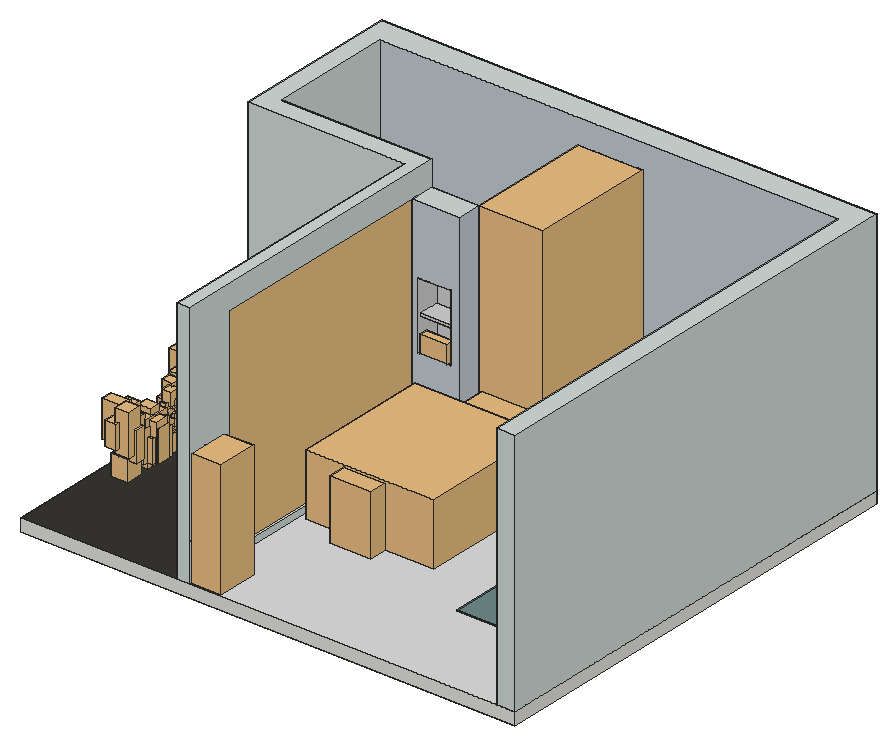
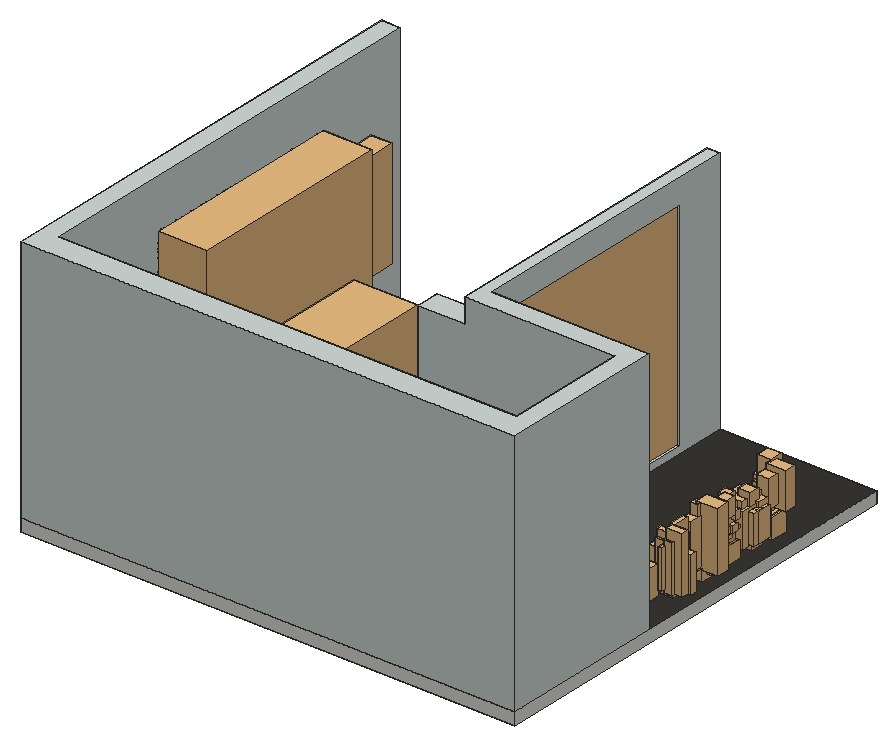
# SketchUp Ruby script. Lengths in inches.
U = 1.inch
M = Sketchup.active_model
def pt(a) = Geom::Point3d.new(a.map { |v| v * U })
def face(e, loops, mat)
  f = e.add_face(loops[0].map { |a| pt(a) })
  loops[1..].each { |l| e.add_face(l.map { |a| pt(a) }).erase! }
  f.material = f.back_material = mat if mat
  f
end
# faces: each face lists its corners as indices into pts; further lists are holes
def faces(e, pts, list, mat = nil) = list.each { |f| face(e, (f[0].is_a?(Array) ? f : [f]).map { |l| l.map { |i| pts[i] } }, mat) }
# xy, xz, yz: faces in a plane at the given z, y or x. An outline is a flat list of corners, or four numbers for a rectangle; further outlines are holes
def ring(l) = l.size == 4 ? [[l[0], l[1]], [l[2], l[1]], [l[2], l[3]], [l[0], l[3]]] : l.each_slice(2).to_a
def flat(e, list, mat, &to3) = list.each { |f| face(e, (f[0].is_a?(Array) ? f : [f]).map { |l| ring(l).map { |u, v| to3.(u, v) } }, mat) }
def xy(e, z, list, mat = nil) = flat(e, list, mat) { |x, y| [x, y, z] }
def xz(e, y, list, mat = nil) = flat(e, list, mat) { |x, z| [x, y, z] }
def yz(e, x, list, mat = nil) = flat(e, list, mat) { |y, z| [x, y, z] }
def lines(e, pts, list) = list.each { |a, b| e.add_line(pt(pts[a]), pt(pts[b])) }
# prism: a flat outline (further loops are holes) pulled along v
def prism(e, loops, v, mat = nil)
  f = face(e, loops, mat); d = Geom::Vector3d.new(v.map { |x| x * U })
  f.pushpull(f.normal.samedirection?(d) ? d.length : -d.length)
end
def box(e, o, s, mat = nil) = prism(e, [[o, [o[0] + s[0], o[1], o[2]], [o[0] + s[0], o[1] + s[1], o[2]], [o[0], o[1] + s[1], o[2]]]], [0, 0, s[2]], mat)
def at(x, y, z, deg = 0) = Geom::Transformation.translation(pt([x, y, z])) * Geom::Transformation.rotation(ORIGIN, Z_AXIS, deg.degrees)
def axes(o, x, y, z) = Geom::Transformation.new([*x, 0, *y, 0, *z, 0, *pt(o).to_a, 1])
def part(name) = M.definitions.add(name)
# library, detail: a bought-in or finely detailed component or shape, given as its bounding box
def library(name, o, s) = part(name).tap { |d| box(d.entities, o, s) }
def detail(e, o, s) = box(e.add_group.entities, o, s)
def put(e, d, t, mat = nil) = e.add_instance(d, t).tap { |i| i.material = mat if mat }
def group(e, t, mat = nil) = e.add_group.tap { |g| g.transformation = t; g.material = mat if mat }.entities
root = M.entities
M.materials.add("1467 AP 9475 Shining Blue").color = [208, 218, 214]
M.materials.add("BANANA_BIG_STVOL_1").color = [93, 83, 53]
M.materials.add("Goldfish-custom-shape__54193.1487305638").color = [111, 138, 137]
M.materials.add("POT_TEXTURE_1").color = [172, 172, 172]
M.materials.add("POT_TEXTURE_2").color = [160, 154, 144]
M.materials.add("[Carrera Marble]").color = [207, 207, 207]
M.materials.add("[Marble Carrara Gold Floor Tile]").color = [221, 221, 221]
M.materials.add("[Metal Seamed]").color = [67, 65, 65]
M.materials.add("[Stone Brushed Khaki]").color = [196, 204, 211]
M.materials.add("[Tile Travertine 2 inch]").color = [56, 54, 50]
M.materials.add("[Translucent Glass Blue]").color = [192, 204, 226]
M.materials["[Translucent Glass Blue]"].alpha = 0.5
M.materials.add("[Wood Floor]").color = [107, 58, 35]
M.materials.add("soil1").color = [68, 55, 47]
M.materials.add("white_concrete_pot1").color = [212, 211, 204]
M.materials.add("wood_1").color = [140, 119, 94]
c1 = library("Сауна. Дренаж",[0,0,0],[36,3.67,1.375])
c2 = library("plant\#1",[-21.34,-27.21,-0.38],[41.91,41.15,38.97])
c3 = library("Untitled",[118.83,25.61,-0.38],[19.68,14.54,56.29])
c4 = library("Group\#283",[-640.625,-1318.37,287.11],[396.64,314.81,689.96])
c5 = library("Group\#277",[-513.94,-1201.2,195.17],[480.66,557.42,1160.08])
c6 = library("Group\#279",[-208.03,-1336.63,286.21],[381.72,484.79,1145.39])
c7 = library("Group\#286",[-619.83,-1636.3,288.9],[316.15,456.61,1171.28])
c8 = library("Group\#287",[-738.91,-1210.08,301],[426.4,388.88,1000.79])
c9 = library("Group\#289",[-208.33,-1511.76,297.04],[508.2,421.96,1258.76])
c10 = library("Group\#278",[-545.36,-1775.03,287.125],[412.21,432,920.68])
c11 = library("Group\#284",[-750.24,-1478.51,301.56],[423.84,451.05,998.69])
c12 = library("Group\#282",[-245.33,-1174.2,301.22],[356.02,306.31,608.34])
c13 = library("Group\#276",[-487.23,-1483.58,-4.71],[450.86,446.99,418.38])
c14 = library("Group\#291",[-445.7,-1606.55,154.18],[255.44,283.57,849.28])
c15 = library("Group\#292",[-390.1,-1177.12,195.59],[220.93,265.44,790.12])
c16 = library("Group\#294",[-480.32,-1333.42,295.8],[424.49,356.06,1482.77])
c17 = library("Group\#295",[-378.01,-1245.98,305.66],[422.15,474.55,1267.42])
c18 = library("Group\#281",[-163.65,-1622.09,292.29],[406.18,374.8,780.12])
c19 = library("Group\#290",[-384.8,-1640.99,300.61],[422.68,348.03,1297.96])
c20 = library("Group\#275",[-429.18,-1441.17,362.05],[345.84,348.28,45.35])
c21 = library("Group\#293",[-208.0625,-1498.77,286.27],[547.26,435.76,1075.6])
c22 = library("Group\#288",[-172.82,-1329.68,294.68],[502.85,397.72,955.79])
c23 = library("Group\#285",[-426.76,-1753.59,287.48],[479.67,412.35,1049.19])
c24 = part("Potted palm")
put(c24.entities,c4,at(750.24,1775.03,4.71))
put(c24.entities,c5,at(750.24,1775.03,4.71))
put(c24.entities,c6,at(750.24,1775.03,4.71))
put(c24.entities,c7,at(750.24,1775.03,4.71))
put(c24.entities,c8,at(750.24,1775.03,4.71))
put(c24.entities,c9,at(750.24,1775.03,4.71))
put(c24.entities,c10,at(750.24,1775.03,4.71))
put(c24.entities,c11,at(750.24,1775.03,4.71))
put(c24.entities,c12,at(750.24,1775.03,4.71))
put(c24.entities,c13,at(750.24,1775.03,4.71),"POT_TEXTURE_1")
put(c24.entities,c14,at(750.24,1775.03,4.71))
put(c24.entities,c15,at(750.24,1775.03,4.71))
put(c24.entities,c16,at(750.24,1775.03,4.71))
put(c24.entities,c17,at(750.24,1775.03,4.71))
put(c24.entities,c18,at(750.24,1775.03,4.71))
put(c24.entities,c19,at(750.24,1775.03,4.71))
put(c24.entities,c20,at(750.24,1775.03,4.71),"soil1")
put(c24.entities,c21,at(750.24,1775.03,4.71))
put(c24.entities,c22,at(750.24,1775.03,4.71))
put(c24.entities,c23,at(750.24,1775.03,4.71))
c25 = library("Scara cu plante",[-7.66,-9.41,-0.15],[30.59,22.83,66.38])
c26 = library("bain4",[0,0,0],[65.98,62.12,30.23])
c27 = library("Group\#14",[0,0,0],[31.13,60.5,108])
c28 = library("Wall hung toilet",[0.42,0,0],[26.94,19.69,42.125])
c29 = part("Goldfish Aqua Runner")
box(c29.entities,[0,0,0],[43.79,100,0.375],"Goldfish-custom-shape__54193.1487305638")
c30 = library("Bathroom Stool and Styling",[15.82,12.47,0],[25.92,25.93,28.18])
c31 = part("Group228\#1")
box(c31.entities,[-18,-24,0],[36,5,0.25])
c32 = part("Group229\#1")
box(c32.entities,[-18,-18.5,0],[36,5,0.25])
c33 = part("Group230\#1")
box(c33.entities,[-18,-13,0],[36,5,0.25])
c34 = part("Group231\#1")
box(c34.entities,[-18,-7.5,0],[36,5,0.25])
c35 = part("Group232\#1")
box(c35.entities,[-18,-2,0],[36,5,0.25])
c36 = part("Group233\#1")
box(c36.entities,[-18,3.5,0],[36,5,0.25])
c37 = part("Group234\#1")
box(c37.entities,[-18,9,0],[36,5,0.25])
c38 = part("Group235\#1")
box(c38.entities,[-18,14.5,0],[36,5,0.25])
c39 = part("Group236\#1")
box(c39.entities,[-18,20,0],[36,4,0.25])
c40 = part("Group226\#1")
put(c40.entities,c31,at(0,0,0))
put(c40.entities,c32,at(0,0,0))
put(c40.entities,c33,at(0,0,0))
put(c40.entities,c34,at(0,0,0))
put(c40.entities,c35,at(0,0,0))
put(c40.entities,c36,at(0,0,0))
put(c40.entities,c37,at(0,0,0))
put(c40.entities,c38,at(0,0,0))
put(c40.entities,c39,at(0,0,0))
c41 = library("Bathroom stool",[0,0,0],[19.9375,11.76,29.04])
c42 = library("Plant\#2",[0,0,0],[12.59,12.59,14.16])
c43 = library("Group\#242",[-662.41,217.3,320.04],[397.32,658.3,1732.06])
c44 = library("Group\#244",[-299.2,181.55,262.58],[360.65,735.71,1258.34])
c45 = library("Group\#239",[-1038.76,656.55,345.34],[733.18,460.51,2065.7])
c46 = library("Group\#237",[-445.29,890.31,329.28],[284.3,304.08,2023.29])
c47 = library("Group\#240",[-733.48,439.625,202.64],[456.28,533.12,1536.78])
c48 = library("Group\#243",[-455.56,899.32,410.78],[341.21,610.33,1581.5])
c49 = library("Group\#236",[-516.34,626.77,-4.5625],[517.73,515.95,418.98])
c50 = library("Group\#241",[-249.24,914.85,310.18],[345.55,647.95,1307.93])
c51 = library("Group\#238",[-277.97,488.68,287.26],[362.84,405.94,1768.54])
c52 = library("Group\#235",[-468.76,669.89,380.1875],[424.36,427.47,41.99])
c53 = part("Potted tropical plant")
put(c53.entities,c43,at(1038.76,-181.55,4.5625))
put(c53.entities,c44,at(1038.76,-181.55,4.5625))
put(c53.entities,c45,at(1038.76,-181.55,4.5625))
put(c53.entities,c46,at(1038.76,-181.55,4.5625))
put(c53.entities,c47,at(1038.76,-181.55,4.5625))
put(c53.entities,c48,at(1038.76,-181.55,4.5625))
put(c53.entities,c49,at(1038.76,-181.55,4.5625),"POT_TEXTURE_1")
put(c53.entities,c50,at(1038.76,-181.55,4.5625))
put(c53.entities,c51,at(1038.76,-181.55,4.5625))
put(c53.entities,c52,at(1038.76,-181.55,4.5625),"soil1")
c54 = library("Group\#248",[-246.45,-349.05,558.47],[136.91,100.49,66.1])
c55 = library("Group\#251",[-264.68,-415.73,1484.11],[304.64,209.69,227.41])
c56 = library("Group\#259",[-357.04,-394.18,1447.05],[213.62,306.36,356.95])
c57 = library("Group\#246",[-447.02,-464.95,536.35],[343.73,346.24,39.39])
c58 = library("Group\#247",[-394.9,-448.99,911.74],[90.19,96.88,85.93])
c59 = library("Group\#258",[-424,-312.27,817.53],[158.81,108.06,136.45])
c60 = library("Group\#262",[-409.02,-515.05,915.53],[69.62,77.27,65.47])
c61 = library("Group\#266",[-548.25,-262.82,1459.54],[373.26,352.35,568])
c62 = library("Group\#274",[-492.14,-508.4,-4.15],[433.72,431.71,567.03])
c63 = library("Group\#269",[-293.78,-482.77,597.9],[158.75,112.78,159.87])
c64 = library("Group\#252",[-545.09,-386.51,922.3125],[300.25,219.65,227.33])
c65 = library("Group\#271",[-292.81,-667.38,1418.14],[215.17,356.07,188.87])
c66 = library("Group\#254",[-292.14,-288.9,1281.79],[169.55,204.34,203.36])
c67 = library("Group\#260",[-568.91,-444.37,1285.4],[307.6,179.39,277.93])
c68 = library("Group\#257",[-341.93,-403.49,744.8125],[64.83,96.32,132.15])
c69 = library("Group\#245",[-258.04,-282.68,604.05],[115.53,137.01,52.63])
c70 = library("Group\#253",[-304.79,-269.16,622.65],[82.06,111.89,102.57])
c71 = library("Group\#261",[-388.93,-514.39,838.93],[89.79,77.73,82.08])
c72 = library("Group\#263",[-295.03,-516.52,742.34],[68.71,141.75,78.67])
c73 = library("Group\#270",[-422.77,-235.4,843.61],[178.54,197.77,233.54])
c74 = library("Group\#264",[-498.98,-524.4,908.45],[120.83,107.95,112.98])
c75 = library("Group\#267",[-321.08,-139.66,1308.49],[285.55,393.29,221.53])
c76 = library("Group\#265",[-278.4,-571.99,1530.91],[311.57,345.77,423.62])
c77 = library("Group\#268",[-387.74,-136.11,1470.07],[230,321.58,230.27])
c78 = library("Group\#256",[-244.55,-305.59,1009.46],[103.13,76.81,77.34])
c79 = library("Group\#273",[-385.21,-446.52,494.02],[160.93,321.12,1142.36])
c80 = library("Group\#249",[-249.18,-250.59,980.93],[152.21,116.16,134.05])
c81 = library("Group\#250",[-438.92,-265.61,702.3],[171.52,146.16,133.5])
c82 = part("Potted houseplant")
p = [[568.91,667.38,4.15],[569.91,667.38,4.15],[569.91,668.38,4.15]]
lines(c82.entities,p,[[0,1],[1,2],[2,0]])
put(c82.entities,c54,at(568.91,667.38,4.15))
put(c82.entities,c55,at(568.91,667.38,4.15))
put(c82.entities,c56,at(568.91,667.38,4.15))
put(c82.entities,c57,at(568.91,667.38,4.15),"soil1")
put(c82.entities,c58,at(568.91,667.38,4.15))
put(c82.entities,c59,at(568.91,667.38,4.15))
put(c82.entities,c60,at(568.91,667.38,4.15))
put(c82.entities,c61,at(568.91,667.38,4.15))
put(c82.entities,c62,at(568.91,667.38,4.15),"POT_TEXTURE_2")
put(c82.entities,c63,at(568.91,667.38,4.15))
put(c82.entities,c64,at(568.91,667.38,4.15))
put(c82.entities,c65,at(568.91,667.38,4.15))
put(c82.entities,c66,at(568.91,667.38,4.15))
put(c82.entities,c67,at(568.91,667.38,4.15))
put(c82.entities,c68,at(568.91,667.38,4.15))
put(c82.entities,c69,at(568.91,667.38,4.15))
put(c82.entities,c70,at(568.91,667.38,4.15))
put(c82.entities,c71,at(568.91,667.38,4.15))
put(c82.entities,c72,at(568.91,667.38,4.15))
put(c82.entities,c73,at(568.91,667.38,4.15))
put(c82.entities,c74,at(568.91,667.38,4.15))
put(c82.entities,c75,at(568.91,667.38,4.15))
put(c82.entities,c76,at(568.91,667.38,4.15))
put(c82.entities,c77,at(568.91,667.38,4.15))
put(c82.entities,c78,at(568.91,667.38,4.15))
put(c82.entities,c79,at(568.91,667.38,4.15),"wood_1")
put(c82.entities,c80,at(568.91,667.38,4.15))
put(c82.entities,c81,at(568.91,667.38,4.15))
c83 = library("Group\#296",[-480.3,-2300.47,677.45],[398.14,398.43,28.25])
c84 = library("Group\#297",[-336.38,-2175.79,614.41],[133.99,147.1,560.64])
c85 = library("Group\#298",[-311.45,-2362.85,663.67],[597.01,322.07,1007.38])
c86 = library("Group\#299",[-330.26,-2159.14,612.04],[116.66,119.22,673.97])
c87 = library("Group\#302",[-667.53,-2111.4375,1071.74],[420.02,555.28,968.03])
c88 = library("Group\#303",[-328.97,-2115.58,1156.29],[117.86,119.42,695.38])
c89 = library("Group\#305",[-943.22,-2312.1875,967.59],[670.63,402.45,1245.73])
c90 = library("Group\#308",[-343.93,-2076.42,1024.91],[285.05,475.82,708.21])
c91 = library("Group\#306",[-568.09,-2386.9,-3.76],[573.62,569.18,700.28])
c92 = library("Group\#309",[-550.09,-2664.39,1031.96],[371.42,533.86,798])
c93 = library("Group\#310",[-308.37,-2556.11,869.35],[483.58,483.6,1385.8])
c94 = part("Potted tropical plant \#1")
put(c94.entities,c83,at(943.22,2664.39,3.76),"soil1")
put(c94.entities,c84,at(943.22,2664.39,3.76),"BANANA_BIG_STVOL_1")
put(c94.entities,c85,at(943.22,2664.39,3.76))
put(c94.entities,c86,at(943.22,2664.39,3.76),"BANANA_BIG_STVOL_1")
put(c94.entities,c87,at(943.22,2664.39,3.76))
put(c94.entities,c88,at(943.22,2664.39,3.76))
put(c94.entities,c89,at(943.22,2664.39,3.76))
put(c94.entities,c90,at(943.22,2664.39,3.76))
put(c94.entities,c91,at(943.22,2664.39,3.76),"POT_TEXTURE_2")
put(c94.entities,c92,at(943.22,2664.39,3.76))
put(c94.entities,c93,at(943.22,2664.39,3.76))
c95 = library("Group\#119",[-312.76,2118.02,370.79],[80.37,61.43,57.53])
c96 = library("Group\#164",[-146.29,2044.53,349.125],[81,53.32,37.9])
c97 = library("Group\#231",[-236.03,2064.57,238.29],[378.97,266.89,1422.96])
c98 = library("Group\#132",[-392.38,2142.99,345.23],[79.77,60.6,39.05])
c99 = library("Group\#193",[-390.04,2074.71,363.78],[77.3,84.83,61.55])
c100 = library("Group\#142",[-389.63,2051.04,359.41],[56.81,81.38,37.86])
c101 = library("Group\#146",[-362.86,1963.26,351.01],[55.56,80.44,37.9])
c102 = library("Group\#163",[-200.52,1998.86,370.22],[77.15,68.38,35.39])
c103 = library("Group\#184",[-480.58,1843.32,11.96],[467.85,466.24,378.92])
c104 = library("Group\#133",[-433.57,2042.61,369.7],[71.79,72.8,37.85])
c105 = library("Group\#130",[-148.5,2084.1,354.63],[73.89,71.73,39.48])
c106 = library("Group\#205",[-372.4375,2154.5,374],[76.125,67.08,39.0625])
c107 = library("Group\#206",[-275.5,2156.34,352.11],[71.39,73.27,44.69])
c108 = library("Group\#174",[-143.56,2061.14,371.42],[79.79,63.19,51.3])
c109 = library("Group\#192",[-363.89,1895.22,354.63],[76.92,66.54,39.48])
c110 = library("Group\#176",[-145.08,2015.32,369.99],[82.29,54.05,37.9])
c111 = library("Group\#203",[-315.77,2202.04,371],[80.74,54.44,37.85])
c112 = library("Group\#194",[-419.21,1941.11,355.02],[73.1,71.21,39.06])
c113 = library("Group\#199",[-229.79,1894.04,351.01],[79.82,63.55,37.9])
c114 = library("Group\#210",[-234.26,2180.97,367.05],[50.63,74.65,43.95])
c115 = library("Group\#213",[-904.81,1865.01,156.3],[624.43,217.34,1227.7])
c116 = library("Group\#214",[-312.51,1611.52,263.78],[120.52,408.52,1275.1])
c117 = library("Group\#217",[-571.16,1736.08,232.33],[294.08,306.57,1438.75])
c118 = library("Group\#222",[-273.21,1593.22,47.51],[374.54,419.07,1416.6])
c119 = library("Group\#123",[-202.35,1900.5,372.29],[58.53,80.11,50.06])
c120 = library("Group\#135",[-432.01,1984.38,372.6875],[64.1,75.95,39.0625])
c121 = library("Group\#168",[-310.7,1952.62,354.63],[79.53,58.52,39.48])
c122 = library("Group\#134",[-374.28,1979.7,369.99],[51.81,82.66,37.9])
c123 = library("Group\#201",[-397.18,1916.74,372.44],[70.02,74.57,49.25])
c124 = library("Group\#208",[-236.3,2186.8,344.47],[79.26,62.91,39.06])
c125 = library("Group\#122",[-161.07,2117.49,373.61],[81.25,53.73,39.48])
c126 = library("Group\#212",[-431.9,1883.46,368.72],[373.65,376.39,18.61])
c127 = library("Group\#167",[-340.96,1970.4,361.28],[81.22,51.59,61.62])
c128 = library("Group\#179",[-272.7,1884.51,369.99],[80.39,55.87,37.9])
c129 = library("Group\#153",[-330.83,2117.69,370.2],[61.83,80.2,35.55])
c130 = library("Group\#209",[-366.3125,2177.8,359.41],[79.9,61.23,37.86])
c131 = library("Group\#145",[-435.875,2067.96,347.82],[58.32,80.53,38.29])
c132 = library("Group\#207",[-183.79,2161.45,371.25],[72.43,70.21,54.35])
c133 = library("Group\#221",[-208.23,2037.18,75.37],[621.09,225.61,1251.82])
c134 = library("Group\#225",[-675.58,1862.05,152.55],[378.81,196.01,1743.84])
c135 = library("Group\#226",[-257.06,2048.08,160.05],[394.6,177.93,1743.83])
c136 = library("Group\#228",[-344.84,1500.61,160.55],[176.35,551.19,1921.45])
c137 = library("Group\#229",[-231.77,1913.24,119.96],[448.93,143.84,1582.05])
c138 = library("Group\#230",[-616.67,2098.6,178.29],[331.19,111.16,1177.92])
c139 = library("Group\#223",[-527.15,2088.47,150.96],[267.01,328.12,1599.25])
c140 = library("Group\#232",[-792.12,2067.32,152.13],[549.56,259.52,1931.8])
c141 = library("Group\#234",[-281.17,2118.67,243.77],[133.23,408.71,1313.3])
c142 = part("Potted houseplant \#1")
g1 = group(c142.entities,at(904.81,-1500.61,-11.96),"white_concrete_pot1")
detail(g1,[-222.14,2117.95,372.07],[61.87,75.41,50.35])
put(c142.entities,c95,at(904.81,-1500.61,-11.96),"white_concrete_pot1")
g2 = group(c142.entities,at(904.81,-1500.61,-11.96),"white_concrete_pot1")
detail(g2,[-313.93,1881.02,351.21],[70.15,73.18,37.2])
g3 = group(c142.entities,at(904.81,-1500.61,-11.96),"white_concrete_pot1")
detail(g3,[-209.1,1970.26,378.89],[50.57,81.04,37.2])
put(c142.entities,c96,at(904.81,-1500.61,-11.96),"white_concrete_pot1")
put(c142.entities,c97,at(904.81,-1500.61,-11.96))
put(c142.entities,c98,at(904.81,-1500.61,-11.96),"white_concrete_pot1")
put(c142.entities,c99,at(904.81,-1500.61,-11.96),"white_concrete_pot1")
put(c142.entities,c100,at(904.81,-1500.61,-11.96),"white_concrete_pot1")
put(c142.entities,c101,at(904.81,-1500.61,-11.96),"white_concrete_pot1")
g4 = group(c142.entities,at(904.81,-1500.61,-11.96),"white_concrete_pot1")
detail(g4,[-129.49,1972.75,359.91],[55.59,80.76,37.2])
put(c142.entities,c102,at(904.81,-1500.61,-11.96),"white_concrete_pot1")
g5 = group(c142.entities,at(904.81,-1500.61,-11.96),"white_concrete_pot1")
detail(g5,[-333.13,1892.25,370.19],[61.39,79.4,37.2])
put(c142.entities,c103,at(904.81,-1500.61,-11.96),"POT_TEXTURE_1")
put(c142.entities,c104,at(904.81,-1500.61,-11.96),"white_concrete_pot1")
put(c142.entities,c105,at(904.81,-1500.61,-11.96),"white_concrete_pot1")
g6 = group(c142.entities,at(904.81,-1500.61,-11.96),"white_concrete_pot1")
detail(g6,[-270.91,2176.57,345.18],[52.11,82.01,38.29])
g7 = group(c142.entities,at(904.81,-1500.61,-11.96),"white_concrete_pot1")
detail(g7,[-195.71,2019.1875,371.11],[58.98,81.18,37.2])
g8 = group(c142.entities,at(904.81,-1500.61,-11.96),"white_concrete_pot1")
detail(g8,[-319.36,2078.81,339.18],[76.07,69.08,39.48])
put(c142.entities,c106,at(904.81,-1500.61,-11.96),"white_concrete_pot1")
put(c142.entities,c107,at(904.81,-1500.61,-11.96),"white_concrete_pot1")
g9 = group(c142.entities,at(904.81,-1500.61,-11.96),"white_concrete_pot1")
detail(g9,[-417.64,2112.53,369.82],[65.44,79.59,38.29])
put(c142.entities,c108,at(904.81,-1500.61,-11.96),"white_concrete_pot1")
put(c142.entities,c109,at(904.81,-1500.61,-11.96),"white_concrete_pot1")
put(c142.entities,c110,at(904.81,-1500.61,-11.96),"white_concrete_pot1")
g10 = group(c142.entities,at(904.81,-1500.61,-11.96),"white_concrete_pot1")
detail(g10,[-240.6,2054.85,378.89],[71.5,72.03,37.2])
put(c142.entities,c111,at(904.81,-1500.61,-11.96),"white_concrete_pot1")
put(c142.entities,c112,at(904.81,-1500.61,-11.96),"white_concrete_pot1")
put(c142.entities,c113,at(904.81,-1500.61,-11.96),"white_concrete_pot1")
g11 = group(c142.entities,at(904.81,-1500.61,-11.96),"white_concrete_pot1")
detail(g11,[-249.82,2117.53,359.91],[58.07,81.25,37.2])
put(c142.entities,c114,at(904.81,-1500.61,-11.96),"white_concrete_pot1")
put(c142.entities,c115,at(904.81,-1500.61,-11.96))
put(c142.entities,c116,at(904.81,-1500.61,-11.96))
put(c142.entities,c117,at(904.81,-1500.61,-11.96))
put(c142.entities,c118,at(904.81,-1500.61,-11.96))
g12 = group(c142.entities,at(904.81,-1500.61,-11.96),"white_concrete_pot1")
detail(g12,[-435.4375,2027.54,350.71],[78.74,62.6,37.86])
put(c142.entities,c119,at(904.81,-1500.61,-11.96),"white_concrete_pot1")
g13 = group(c142.entities,at(904.81,-1500.61,-11.96),"white_concrete_pot1")
detail(g13,[-173.8,2126.25,354.63],[80.17,60.53,39.48])
g14 = group(c142.entities,at(904.81,-1500.61,-11.96),"white_concrete_pot1")
detail(g14,[-222.96,2066.75,359.91],[63.77,78.21,37.2])
put(c142.entities,c120,at(904.81,-1500.61,-11.96),"white_concrete_pot1")
g15 = group(c142.entities,at(904.81,-1500.61,-11.96),"white_concrete_pot1")
detail(g15,[-183.125,1913.38,330.04],[66.78,77.69,39.48])
put(c142.entities,c121,at(904.81,-1500.61,-11.96),"white_concrete_pot1")
g16 = group(c142.entities,at(904.81,-1500.61,-11.96),"white_concrete_pot1")
detail(g16,[-152,1936.85,378.89],[64.46,79.76,37.2])
g17 = group(c142.entities,at(904.81,-1500.61,-11.96),"white_concrete_pot1")
detail(g17,[-284.65,1933.22,373.64],[80.83,55.23,37.2])
put(c142.entities,c122,at(904.81,-1500.61,-11.96),"white_concrete_pot1")
g18 = group(c142.entities,at(904.81,-1500.61,-11.96),"white_concrete_pot1")
detail(g18,[-263.49,1923.54,359.91],[75.98,66.75,37.2])
put(c142.entities,c123,at(904.81,-1500.61,-11.96),"white_concrete_pot1")
g19 = group(c142.entities,at(904.81,-1500.61,-11.96),"white_concrete_pot1")
detail(g19,[-167.97,1940.97,354.63],[66.78,77.7,39.48])
put(c142.entities,c124,at(904.81,-1500.61,-11.96),"white_concrete_pot1")
g20 = group(c142.entities,at(904.81,-1500.61,-11.96),"white_concrete_pot1")
detail(g20,[-214.75,1956.59,330.04],[66.78,77.69,39.48])
put(c142.entities,c125,at(904.81,-1500.61,-11.96),"white_concrete_pot1")
put(c142.entities,c126,at(904.81,-1500.61,-11.96),"white_concrete_pot1")
put(c142.entities,c127,at(904.81,-1500.61,-11.96),"white_concrete_pot1")
g21 = group(c142.entities,at(904.81,-1500.61,-11.96),"white_concrete_pot1")
detail(g21,[-282.5625,1934.21,389.56],[81.1,59.19,35.03])
put(c142.entities,c128,at(904.81,-1500.61,-11.96),"white_concrete_pot1")
g22 = group(c142.entities,at(904.81,-1500.61,-11.96),"white_concrete_pot1")
detail(g22,[-394.5,2036.48,359.91],[79.58,64.84,37.2])
put(c142.entities,c129,at(904.81,-1500.61,-11.96),"white_concrete_pot1")
put(c142.entities,c130,at(904.81,-1500.61,-11.96),"white_concrete_pot1")
put(c142.entities,c131,at(904.81,-1500.61,-11.96),"white_concrete_pot1")
put(c142.entities,c132,at(904.81,-1500.61,-11.96),"white_concrete_pot1")
put(c142.entities,c133,at(904.81,-1500.61,-11.96))
put(c142.entities,c134,at(904.81,-1500.61,-11.96))
put(c142.entities,c135,at(904.81,-1500.61,-11.96))
put(c142.entities,c136,at(904.81,-1500.61,-11.96))
put(c142.entities,c137,at(904.81,-1500.61,-11.96))
put(c142.entities,c138,at(904.81,-1500.61,-11.96))
put(c142.entities,c139,at(904.81,-1500.61,-11.96))
put(c142.entities,c140,at(904.81,-1500.61,-11.96))
put(c142.entities,c141,at(904.81,-1500.61,-11.96))
c143 = library("Group\#16",[-0.5,0,0],[3,114,105])
c144 = part("Group\#18")
box(c144.entities,[-0.47,0,0],[0.47,56,101])
c145 = library("Group\#5",[-20.5,-2,0],[20.5,100,87])
c146 = library("Wall Tap 1",[0,0,0],[12.6,7.22,3.6875])
c147 = library("JEE-O slimline shower set bronze\#1",[0.04,-0.03,-18.98],[11.61,24.11,65.69])
c148 = library("Bathrobe with hooks",[0,0,-0.08],[18.125,10.02,52.34])
c149 = library("Group\#52",[0,-0.31,0],[12.93,3.92,8.58])
xy(root,0,[[76,0,76,138,0,138,0,219,240,219,240,0,231,0,231,147,195,147,195,153,231,153,231,207,9,207,9,147,105,147,105,135,82,135,82,0]],"1467 AP 9475 Shining Blue")
xy(root,3,[[76,24,82,138]],"1467 AP 9475 Shining Blue")
xy(root,42,[[85,135,101,146]],"[Carrera Marble]")
xy(root,48,[[195,147,231,153]],"1467 AP 9475 Shining Blue")
xy(root,48,[[50.5,207,110.5,213]],"[Carrera Marble]")
xy(root,58,[[85,145,101,146]],"1467 AP 9475 Shining Blue")
xy(root,58,[[85,136,101,144]],"[Carrera Marble]")
xy(root,58.5,[[85,144,101,145]],"1467 AP 9475 Shining Blue")
xy(root,59,[[85,136,101,146]],"[Carrera Marble]")
xy(root,63,[[50.5,207,110.5,211],[50.5,212,110.5,213]],"1467 AP 9475 Shining Blue")
xy(root,63.5,[[50.5,211,110.5,212]],"1467 AP 9475 Shining Blue")
xy(root,75,[[85,135,101,144],[85,145,101,146]],"1467 AP 9475 Shining Blue")
xy(root,75.5,[[85,144,101,145]],"1467 AP 9475 Shining Blue")
xy(root,108,[[76,24,82,138],[82,135,105,147]],"1467 AP 9475 Shining Blue")
xy(root,120,[[76,0,82,0,82,147,9,147,9,207,231,207,231,0,240,0,240,219,0,219,0,138,76,138]],"1467 AP 9475 Shining Blue")
xz(root,0,[[76,0,82,120],[231,0,240,120]],"1467 AP 9475 Shining Blue")
xz(root,24,[[76,3,82,108]],"1467 AP 9475 Shining Blue")
xz(root,135,[[[82,0,105,108],[85,42,101,75]]],"[Stone Brushed Khaki]")
xz(root,136,[[85,58,101,59]],"[Carrera Marble]")
xz(root,138,[[0,0,76,0,76,3,82,3,82,108,76,108,76,120,0,120]],"1467 AP 9475 Shining Blue")
xz(root,144,[[85,58,101,58.5],[85,75,101,75.5]],"1467 AP 9475 Shining Blue")
xz(root,145,[[85,58,101,58.5],[85,75,101,75.5]],"1467 AP 9475 Shining Blue")
xz(root,146,[[85,42,101,58],[85,59,101,75]],"[Carrera Marble]")
xz(root,147,[[9,0,9,120,82,120,82,108,105,108,105,0],[195,0,231,48]],"1467 AP 9475 Shining Blue")
xz(root,153,[[195,0,231,48]],"1467 AP 9475 Shining Blue")
xz(root,207,[[[9,0,231,120],[50.5,48,110.5,63]]],"[Stone Brushed Khaki]")
xz(root,211,[[50.5,63,110.5,63.5]],"1467 AP 9475 Shining Blue")
xz(root,212,[[50.5,63,110.5,63.5]],"1467 AP 9475 Shining Blue")
xz(root,213,[[50.5,48,110.5,63]],"[Carrera Marble]")
xz(root,219,[[0,0,240,120]],"1467 AP 9475 Shining Blue")
yz(root,0,[[138,0,219,120]],"1467 AP 9475 Shining Blue")
yz(root,9,[[147,0,207,120]],"1467 AP 9475 Shining Blue")
yz(root,50.5,[[207,48,213,48,213,63,212,63,212,63.5,211,63.5,211,63,207,63]],"1467 AP 9475 Shining Blue")
yz(root,76,[[0,0,0,120,138,120,138,108,24,108,24,3,138,3,138,0]],"1467 AP 9475 Shining Blue")
yz(root,82,[[0,0,135,0,135,3,24,3,24,108,147,108,147,120,0,120],[135,3,138,108]],"1467 AP 9475 Shining Blue")
yz(root,85,[[135,42,146,42,146,58,145,58,145,58.5,144,58.5,144,58,136,58,136,59,146,59,146,75,145,75,145,75.5,144,75.5,144,75,135,75]],"[Carrera Marble]")
yz(root,101,[[135,42,135,75,144,75,144,75.5,145,75.5,145,75,146,75,146,59,136,59,136,58,144,58,144,58.5,145,58.5,145,58,146,58,146,42]],"[Carrera Marble]")
yz(root,105,[[135,0,147,108]],"[Stone Brushed Khaki]")
yz(root,110.5,[[207,48,207,63,211,63,211,63.5,212,63.5,212,63,213,63,213,48]],"[Carrera Marble]")
yz(root,195,[[147,0,153,48]],"1467 AP 9475 Shining Blue")
yz(root,231,[[0,0,0,120,207,120,207,0,153,0,153,48,147,48,147,0]],"1467 AP 9475 Shining Blue")
yz(root,240,[[0,0,219,120]],"1467 AP 9475 Shining Blue")
g23 = group(root,at(57,0,0))
xy(g23,-6,[[-57,0,183,219]])
xy(g23,-1,[[47.96,201.875,68.48,203.97]])
xy(g23,0,[[[19,0,183,0,183,219,-57,219,-57,138,19,138],[47.96,201.875,68.48,203.97]]],"[Marble Carrara Gold Floor Tile]")
xy(g23,0,[[-57,0,19,138]],"[Tile Travertine 2 inch]")
xz(g23,0,[[-57,-6,183,0]])
xz(g23,201.875,[[47.96,-1,68.48,0]])
xz(g23,203.97,[[47.96,-1,68.48,0]])
xz(g23,219,[[-57,-6,183,0]])
yz(g23,-57,[[0,-6,219,0]])
yz(g23,47.96,[[201.875,-1,203.97,0]])
yz(g23,68.48,[[201.875,-1,203.97,0]])
yz(g23,183,[[0,-6,219,0]])
p = [[25,0,0],[25,135,0]]
lines(g23,p,[[0,1]])
put(g23,c1,axes([47.96,201.875,-0.78],[0.57,0,0],[0,0.57,0],[0,0,0.57]))
put(root,c2,at(47.16,127.24,0,-60),"1467 AP 9475 Shining Blue")
put(root,c3,axes([122.15,139.56,0.38],[0,-1,0],[-1,0,0],[0,0,1]),"1467 AP 9475 Shining Blue")
put(root,c24,axes([4.09,55.33,0],[0.01419,0,0],[0,0.01419,0],[0,0,0.01419]),"1467 AP 9475 Shining Blue")
put(root,c25,at(53.07,124.5625,0.15),"1467 AP 9475 Shining Blue")
put(root,c26,axes([147.1875,132.68,0],[0,-1,0],[-1,0,0],[0,0,1]),"1467 AP 9475 Shining Blue")
put(root,c27,at(105,146.5,0),"1467 AP 9475 Shining Blue")
put(root,c28,at(231,167.95,0,90),"1467 AP 9475 Shining Blue")
put(root,c29,axes([174.33,47,0],[0.93,0,0],[0,1,0],[0,0,1]),"1467 AP 9475 Shining Blue")
put(root,c30,at(90.98,111.53,0),"1467 AP 9475 Shining Blue")
put(root,c40,axes([213,147,24],[1,0,0],[0,0,1],[0,-1,0]),"[Wood Floor]")
put(root,c41,at(103.66,58.09,0),"1467 AP 9475 Shining Blue")
put(root,c42,at(13.72,115.57,0),"1467 AP 9475 Shining Blue")
put(root,c53,axes([0,83.09,0],[0.01419,0,0],[0,0.01419,0],[0,0,0.01419]),"1467 AP 9475 Shining Blue")
put(root,c82,axes([6.67,71.05,0.01],[0.01419,0,0],[0,0.01419,0],[0,0,0.01419]),"1467 AP 9475 Shining Blue")
put(root,c94,axes([1.36,42.71,0.01],[0.01419,0,0],[0,0.01419,0],[0,0,0.01419]),"1467 AP 9475 Shining Blue")
put(root,c142,axes([1.9,101.81,0.24],[0.01419,0,0],[0,0.01419,0],[0,0,0.01419]),"1467 AP 9475 Shining Blue")
g24 = group(root,at(78,24,3),"[Metal Seamed]")
put(g24,c143,at(0,0,0))
g25 = group(g24,at(0.09,2.93,1))
xy(g25,-0.3,[[0.09,53.07,0.28,110.07],[0.41,53.07,0.72,110.07]])
xy(g25,0,[[0.28,52.82,0.41,109.82],[0,53.07,0.09,110.07],[0.72,53.07,0.8125,110.07]])
xy(g25,1,[[0,54.05,0.8125,109.09]])
xy(g25,102,[[0,54.05,0.8125,109.09]])
xy(g25,103,[[0.28,52.82,0.41,109.82],[0,53.07,0.09,110.07],[0.72,53.07,0.8125,110.07]])
xy(g25,103.3,[[0.09,53.07,0.28,110.07],[0.41,53.07,0.72,110.07]])
xz(g25,52.82,[[0.28,0,0.41,103]])
xz(g25,53.07,[[0.09,-0.3,0.28,-0.3,0.28,103.3,0.09,103.3,0.09,103,0,103,0,0,0.09,0],[0.41,-0.3,0.72,-0.3,0.72,0,0.8125,0,0.8125,103,0.72,103,0.72,103.3,0.41,103.3]])
xz(g25,54.05,[[0,1,0.8125,102]])
xz(g25,109.09,[[0,1,0.8125,102]])
xz(g25,109.82,[[0.28,0,0.41,103]])
xz(g25,110.07,[[0.09,-0.3,0.09,0,0,0,0,103,0.09,103,0.09,103.3,0.28,103.3,0.28,-0.3],[0.41,-0.3,0.41,103.3,0.72,103.3,0.72,103,0.8125,103,0.8125,0,0.72,0,0.72,-0.3]])
yz(g25,0,[[[53.07,0,110.07,103],[54.05,1,109.09,102]]])
yz(g25,0.09,[[53.07,-0.3,110.07,0],[53.07,103,110.07,103.3]])
yz(g25,0.28,[[53.07,-0.3,109.82,0],[109.82,-0.3,110.07,103.3],[52.82,0,53.07,103],[53.07,103,53.31,103.3],[53.31,103,109.82,103.3]])
yz(g25,0.41,[[53.07,-0.3,109.82,0],[109.82,-0.3,110.07,103.3],[52.82,0,53.07,103],[53.07,103,53.31,103.3],[53.31,103,109.82,103.3]])
yz(g25,0.72,[[53.07,-0.3,110.07,0],[53.07,103,110.07,103.3]])
yz(g25,0.8125,[[[53.07,0,110.07,103],[54.05,1,109.09,102]]])
p = [[0.28,53.31,103],[0.09,110.07,103],[-0.09,109.09,1],[0,109.09,102],[0,54.05,1]]
lines(g25,p,[[0,1],[2,3],[4,2]])
put(g25,c144,axes([0.68,54.05,1],[1,0,0],[0,0.98276,0],[0,0,1]),"[Translucent Glass Blue]")
g26 = group(g24,at(1.91,-52.07,1))
xy(g26,-0.3,[[-0.72,53.07,-0.41,110.07],[-0.28,53.07,-0.09,110.07]])
xy(g26,0,[[-0.8125,53.07,-0.72,110.07],[-0.09,53.07,0,110.07],[-0.41,53.31,-0.28,109.82]])
xy(g26,1,[[-0.8125,54.05,0,109.09]])
xy(g26,102,[[-0.8125,54.05,0,109.09]])
xy(g26,103,[[-0.8125,53.07,-0.72,110.07],[-0.09,53.07,0,110.07],[-0.41,53.31,-0.28,109.82]])
xy(g26,103.3,[[-0.72,53.07,-0.41,110.07],[-0.28,53.07,-0.09,110.07]])
xz(g26,53.07,[[-0.72,-0.3,-0.72,0,-0.8125,0,-0.8125,103,-0.72,103,-0.72,103.3,-0.41,103.3,-0.41,-0.3],[-0.28,-0.3,-0.28,103.3,-0.09,103.3,-0.09,103,0,103,0,0,-0.09,0,-0.09,-0.3]])
xz(g26,53.31,[[-0.41,0,-0.28,103]])
xz(g26,54.05,[[-0.8125,1,0,102]])
xz(g26,109.09,[[-0.8125,1,0,102]])
xz(g26,109.82,[[-0.41,0,-0.28,103]])
xz(g26,110.07,[[-0.72,-0.3,-0.41,-0.3,-0.41,103.3,-0.72,103.3,-0.72,103,-0.8125,103,-0.8125,0,-0.72,0],[-0.28,-0.3,-0.09,-0.3,-0.09,0,0,0,0,103,-0.09,103,-0.09,103.3,-0.28,103.3]])
yz(g26,-0.8125,[[[53.07,0,110.07,103],[54.05,1,109.09,102]]])
yz(g26,-0.72,[[53.07,-0.3,110.07,0],[53.07,103,110.07,103.3]])
yz(g26,-0.41,[[53.07,-0.3,53.07,103.3,53.31,103.3,53.31,0,109.82,0,109.82,-0.3],[109.82,-0.3,110.07,103.3],[53.31,103,109.82,103.3]])
yz(g26,-0.28,[[53.07,-0.3,109.82,-0.3,109.82,0,53.31,0,53.31,103,53.07,103],[109.82,-0.3,110.07,103.3],[53.07,103,53.31,103.3],[53.31,103,109.82,103.3]])
yz(g26,-0.09,[[53.07,-0.3,110.07,0],[53.07,103,110.07,103.3]])
yz(g26,0,[[[53.07,0,110.07,103],[54.05,1,109.09,102]]])
p = [[-0.28,53.31,103],[-0.09,110.07,103]]
lines(g26,p,[[0,1]])
put(g26,c144,axes([-0.68,54.05,1],[-1,0,0],[0,0.98276,0],[0,0,1]),"[Translucent Glass Blue]")
put(root,c145,axes([231,49,9],[1.17073,0,0],[0,1,0],[0,0,1]),"1467 AP 9475 Shining Blue")
g27 = group(root,at(45,207,18),"1467 AP 9475 Shining Blue")
xy(g27,-2,[[12,-10,14,0],[34,-10,36,0]])
xy(g27,0,[[0,-15,0,0,12,0,12,-10,14,-10,14,0,34,0,34,-10,36,-10,36,0,48,0,48,-15]])
xy(g27,2,[[0,-15,48,0]])
xz(g27,-15,[[0,0,48,2]])
xz(g27,-10,[[12,-2,14,0],[34,-2,36,0]])
xz(g27,0,[[12,-2,12,0,0,0,0,2,48,2,48,0,36,0,36,-2,34,-2,34,0,14,0,14,-2]])
yz(g27,0,[[-15,0,0,2]])
yz(g27,12,[[-10,-2,0,0]])
yz(g27,14,[[-10,-2,0,0]])
yz(g27,34,[[-10,-2,0,0]])
yz(g27,36,[[-10,-2,0,0]])
yz(g27,48,[[-15,0,0,2]])
put(root,c146,axes([78.31,154.22,24],[1,0,0],[0,-1,0],[0,0,1]),"1467 AP 9475 Shining Blue")
put(root,c147,axes([115.35,182.92,40.89],[0.89,0,0],[0,0.89,0],[0,0,0.89]),"1467 AP 9475 Shining Blue")
put(root,c148,at(231,17.85,28.74,92.5),"1467 AP 9475 Shining Blue")
put(root,c149,axes([98.83,135.31,42],[-1,0,0],[0,1,0],[0,0,1]))
